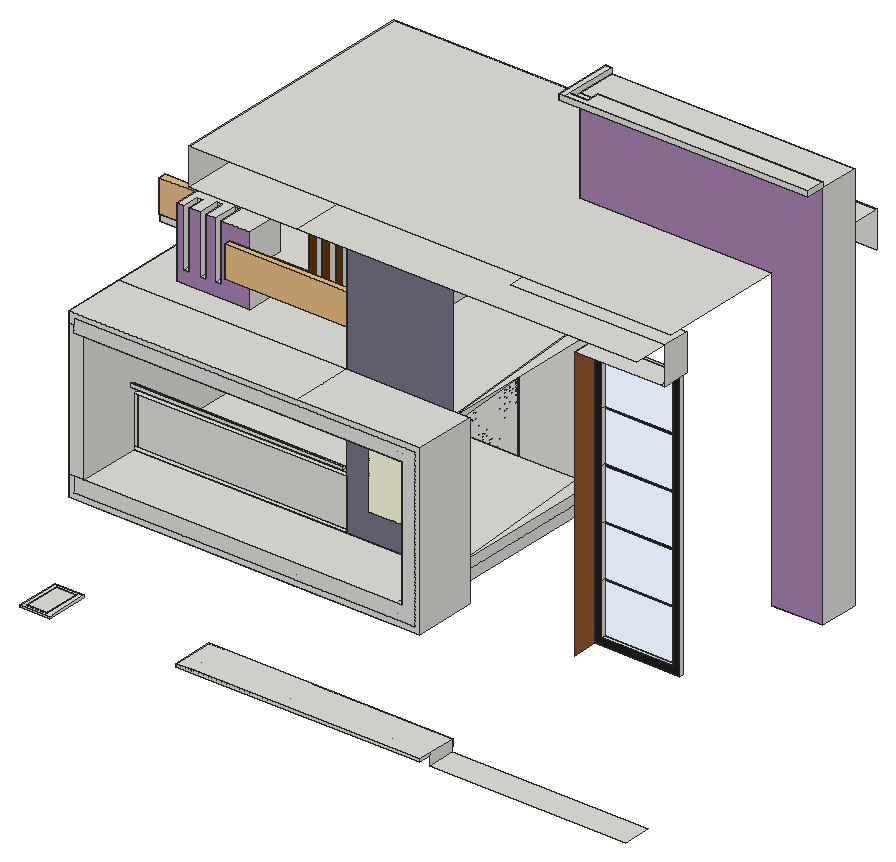
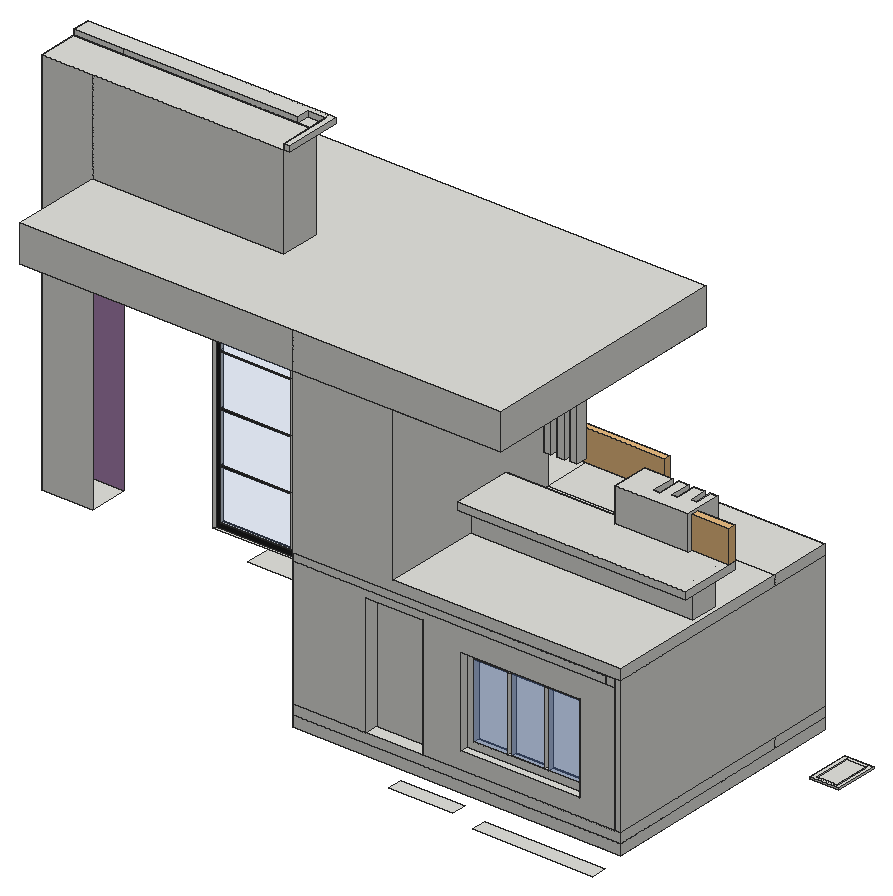
# SketchUp Ruby script. Lengths in inches.
U = 1.inch
M = Sketchup.active_model
def pt(a) = Geom::Point3d.new(a.map { |v| v * U })
def face(e, loops, mat)
  f = e.add_face(loops[0].map { |a| pt(a) })
  loops[1..].each { |l| e.add_face(l.map { |a| pt(a) }).erase! }
  f.material = f.back_material = mat if mat
  f
end
# faces: each face lists its corners as indices into pts; further lists are holes
def faces(e, pts, list, mat = nil) = list.each { |f| face(e, (f[0].is_a?(Array) ? f : [f]).map { |l| l.map { |i| pts[i] } }, mat) }
# xy, xz, yz: faces in a plane at the given z, y or x. An outline is a flat list of corners, or four numbers for a rectangle; further outlines are holes
def ring(l) = l.size == 4 ? [[l[0], l[1]], [l[2], l[1]], [l[2], l[3]], [l[0], l[3]]] : l.each_slice(2).to_a
def flat(e, list, mat, &to3) = list.each { |f| face(e, (f[0].is_a?(Array) ? f : [f]).map { |l| ring(l).map { |u, v| to3.(u, v) } }, mat) }
def xy(e, z, list, mat = nil) = flat(e, list, mat) { |x, y| [x, y, z] }
def xz(e, y, list, mat = nil) = flat(e, list, mat) { |x, z| [x, y, z] }
def yz(e, x, list, mat = nil) = flat(e, list, mat) { |y, z| [x, y, z] }
def lines(e, pts, list) = list.each { |a, b| e.add_line(pt(pts[a]), pt(pts[b])) }
# prism: a flat outline (further loops are holes) pulled along v
def prism(e, loops, v, mat = nil)
  f = face(e, loops, mat); d = Geom::Vector3d.new(v.map { |x| x * U })
  f.pushpull(f.normal.samedirection?(d) ? d.length : -d.length)
end
def box(e, o, s, mat = nil) = prism(e, [[o, [o[0] + s[0], o[1], o[2]], [o[0] + s[0], o[1] + s[1], o[2]], [o[0], o[1] + s[1], o[2]]]], [0, 0, s[2]], mat)
def at(x, y, z, deg = 0) = Geom::Transformation.translation(pt([x, y, z])) * Geom::Transformation.rotation(ORIGIN, Z_AXIS, deg.degrees)
def axes(o, x, y, z) = Geom::Transformation.new([*x, 0, *y, 0, *z, 0, *pt(o).to_a, 1])
def part(name) = M.definitions.add(name)
# library, detail: a bought-in or finely detailed component or shape, given as its bounding box
def library(name, o, s) = part(name).tap { |d| box(d.entities, o, s) }
def detail(e, o, s) = box(e.add_group.entities, o, s)
def put(e, d, t, mat = nil) = e.add_instance(d, t).tap { |i| i.material = mat if mat }
def group(e, t, mat = nil) = e.add_group.tap { |g| g.transformation = t; g.material = mat if mat }.entities
root = M.entities
M.materials.add("Ston e Marble").color = [119, 117, 136]
M.materials.add("[0054_LightYellow]").color = [255, 255, 224]
M.materials.add("[0126_Violet]").color = [168, 130, 177]
M.materials.add("[Color C08]").color = [102, 51, 0]
M.materials.add("[Color L02]").color = [190, 153, 204]
M.materials.add("[Color M08]").color = [30, 30, 30]
M.materials.add("[Translucent Glass Blue]").color = [100, 146, 237]
M.materials["[Translucent Glass Blue]"].alpha = 0.42
M.materials.add("[Translucent Glass Blue]2").color = [100, 149, 237]
M.materials["[Translucent Glass Blue]2"].alpha = 0.01
M.materials.add("[Translucent Glass Blue]3").color = [100, 149, 237]
M.materials["[Translucent Glass Blue]3"].alpha = 0.2
M.materials.add("[Wood Cherry Original]").color = [152, 86, 42]
c1 = part("DOOR12")
g1 = group(c1.entities,at(114.73,28.14,-0.51))
g2 = group(g1,at(0,0,0))
box(g2,[0,0,0],[36,0.5,77.7])
c2 = part("Group\#1")
xy(c2.entities,0,[[0,0,74.375,3.6875]])
xy(c2.entities,4.39,[[4.39,0,24.03,3.6875],[24.03,0,26.53,3.6875],[26.53,0,47.01,3.6875],[47.01,0,49.38,3.6875],[49.38,0,69.98,3.6875]])
xy(c2.entities,50.55,[[4.39,0,24.03,3.6875],[24.03,0,26.53,3.6875],[26.53,0,47.01,3.6875],[47.01,0,49.38,3.6875],[49.38,0,69.98,3.6875]])
xy(c2.entities,54.9375,[[0,0,74.375,3.6875]])
xz(c2.entities,0,[[[0,0,74.375,54.9375],[4.39,4.39,69.98,50.55]],[24.03,4.39,26.53,50.55],[47.01,4.39,49.38,50.55]],"[Color M08]")
xz(c2.entities,3.6875,[[[0,0,74.375,54.9375],[4.39,4.39,69.98,50.55]]])
xz(c2.entities,3.6875,[[4.39,4.39,24.03,50.55],[26.53,4.39,47.01,50.55],[49.38,4.39,69.98,50.55]],"[Translucent Glass Blue]")
yz(c2.entities,0,[[0,0,3.6875,54.9375]])
yz(c2.entities,4.39,[[0,4.39,3.6875,50.55]])
yz(c2.entities,24.03,[[0,4.39,3.6875,50.55]])
yz(c2.entities,26.53,[[0,4.39,3.6875,50.55]])
yz(c2.entities,47.01,[[0,4.39,3.6875,50.55]])
yz(c2.entities,49.38,[[0,4.39,3.6875,50.55]])
yz(c2.entities,69.98,[[0,4.39,3.6875,50.55]])
yz(c2.entities,74.375,[[0,0,3.6875,54.9375]])
c3 = library("Group\#4",[0,0,0],[173.05,8.28,46.41])
xy(root,38.6875,[[252.01,49.71,373.22,66.43]])
xy(root,38.8125,[[165.8,49.71,197.22,67.24]])
xy(root,41.375,[[228.64,66.43,252.01,67.24]])
xy(root,42.6875,[[[4.76,42.32,22.75,69],[7.2,44,19.58,67.25]]])
xy(root,43.9375,[[101.44,41.71,101.44,67.24,110.38,67.24,110.38,49.71,252.01,49.71,252.01,41.71],[[4.76,42.32,22.75,69],[7.2,44,19.58,67.25]],[7.2,44,19.58,67.25]])
xy(root,45.75,[[101.44,41.71,252.01,67.24]])
xy(root,66.45,[[18,233.8,92.38,242.8]])
xy(root,71.33,[[104.9375,233.8,144.61,242.8]])
xy(root,84,[[1.2,84.18,10.2,122.8],[10.2,84.18,10.2,233.8,195.57,233.8,195.57,122.8,142,122.8,142,84.18],[142,84.18,195.57,122.8],[195.57,84.18,204.07,122.8],[204.07,84.18,218.2,122.8],
  [1.2,122.8,10.2,242.8],[195.57,122.8,204.07,233.8],[10.2,233.8,204.07,242.8]])
xy(root,90.65,[[1.2,122.8,204.07,242.8]])
xy(root,90.8125,[[296.76,120.86,349.59,122.8]])
xy(root,95.41,[[301.36,120.86,344.99,122.8]])
xy(root,96.65,[[1.2,84.18,10.42,122.8],[10.42,84.18,204.07,122.8],[1.2,122.8,4.42,122.8,4.42,125.91,10.42,125.91,10.42,233.8,4.42,233.8,4.42,242.8,1.2,242.8],[142,122.8,204.07,122.8,195.57,233.8,10.42,233.8,10.42,125.91,142,125.91],[204.07,122.8,195.57,233.8,204.07,233.8],
  [4.42,233.8,123.41,242.8],[123.41,233.8,159.14,242.8],[159.14,233.8,204.07,242.8]])
xy(root,107.12,[[26.05,233.8,100.42,242.8]])
xy(root,120.43,[[373.22,162.34,404.66,186.78]])
xy(root,128.03,[[4.42,122.8,10.42,125.91],[10.42,122.8,142,125.91]])
xy(root,162.05,[[26.05,233.8,100.42,242.8]])
xy(root,171.64,[[123.41,233.8,159.14,242.8]])
xy(root,176.09,[[10.42,84.18,10.42,233.8,195.57,233.8,204.07,122.8,204.07,84.18],[204.07,84.18,207.2,122.8],[4.42,122.8,10.2,233.8],[10.2,122.8,10.42,233.8],[4.42,233.8,10.2,242.8],
  [10.2,233.8,204.07,242.8]])
xy(root,180.65,[[1.2,84.18,4.42,122.8],[1.2,122.8,4.42,242.8],[4.42,122.8,10.2,242.8],[204.07,122.8,204.07,233.8,195.57,233.8],[10.2,233.8,204.07,242.8]])
xy(root,187.31,[[1.2,84.18,142,122.8],[142,84.18,218.2,122.8],[[1.2,122.8,142,122.8,142,165.79,4.26,165.79,4.26,182.8,142,182.8,142,242.8,1.2,242.8],[23.57,139.58,68.88,162.39]]])
xy(root,194.74,[[28.08,139.58,31.21,149.83]])
xy(root,194.87,[[38.29,139.58,41.54,152.26]])
xy(root,195.12,[[47.72,139.58,51.1,154.2]])
xy(root,204.87,[[0,155.96,4.26,165.79],[4.26,155.96,142,165.79],[0,165.79,4.26,182.8],[0,182.8,4.26,193.76],[4.26,182.8,142,193.76]])
xy(root,209.43,[[0,155.96,142,193.76]])
xy(root,219.41,[[108.41,135.83,113.16,142.39],[115.68,136.58,120.68,143.02],[124.125,136.68,128.8125,142.99]])
xy(root,230.31,[[23.57,139.58,28.08,139.58,28.08,149.83,31.21,149.83,31.21,139.58,38.29,139.58,38.29,152.26,41.54,152.26,41.54,139.58,47.72,139.58,47.72,154.2,51.1,154.2,51.1,139.58,68.88,139.58,68.88,162.39,23.57,162.39]])
xy(root,254.35,[[301.36,120.86,344.99,122.8]])
xy(root,258.95,[[296.76,105.55,349.59,120.86],[349.59,105.55,352.27,122.8],[296.76,120.86,349.59,122.8]])
xy(root,282.04,[[[75.43,84.18,142,242.8],[115.68,136.58,120.68,143.02],[108.41,135.83,113.16,142.39],[124.125,136.68,128.8125,142.99]],[142,84.18,142,122.8,256.63,122.8,256.63,105.55,352.27,105.55,352.27,84.18],[256.63,105.55,352.27,122.8]])
xy(root,304.31,[[75.43,84.18,373.22,84.18,373.22,162.34,254.66,162.34,254.66,186.78,373.22,186.78,373.22,242.8,75.43,242.8]])
xy(root,362.43,[[250.79,150.97,254.66,186.78],[254.66,150.97,404.66,150.97,404.66,162.34,265.51,162.34,265.51,154.47,254.66,154.47],[254.66,154.47,265.51,162.34],[254.66,162.34,404.66,186.78]])
xy(root,365.68,[[250.79,150.97,254.66,186.78],[254.66,150.97,404.66,150.97,404.66,162.34,265.51,162.34,265.51,154.47,254.66,154.47]])
xz(root,41.71,[[101.44,43.9375,110.38,45.75],[110.38,43.9375,252.01,45.75]])
xz(root,42.32,[[4.76,42.6875,22.75,43.9375]])
xz(root,44,[[7.2,42.6875,19.58,43.9375]])
xz(root,49.71,[[197.22,38.5625,228.64,38.5625,228.64,43.9375,165.8,43.9375,165.8,38.8125,197.22,38.8125]],"[Color L02]")
xz(root,67.24,[[165.8,38.8125,165.8,45.75,252.01,45.75,252.01,41.375,197.22,41.375,197.22,38.8125],[101.44,43.9375,110.38,45.75]])
xz(root,67.25,[[7.2,42.6875,19.58,43.9375]])
xz(root,69,[[4.76,42.6875,22.75,43.9375]])
xz(root,84.18,[[1.2,84,218.2,84,218.2,187.31,1.2,187.31,1.2,180.65,4.42,180.65,4.42,184.09,214.98,184.09,214.98,87.22,4.42,87.22,4.42,96.65,1.2,96.65],[4.42,87.22,214.98,87.22,214.98,184.09,4.42,184.09,4.42,176.09,207.2,176.09,207.2,96.59,204.07,96.65,4.42,96.65],[1.2,96.65,10.42,96.65,10.42,176.09,4.42,176.09,4.42,180.65,1.2,180.65]])
xz(root,119.85,[[10.42,132.73,142,134.54]])
xz(root,120.86,[[[296.76,90.8125,349.59,258.95],[301.36,95.41,344.99,254.35]]],"[Color M08]")
xz(root,121.36,[[10.42,132.75,142,134.56]])
xz(root,122.8,[[142,84,204.07,90.65],[204.07,84,218.2,90.65],[1.2,90.65,142,96.65],[142,90.65,204.07,96.65],[204.07,90.65,204.07,96.65,207.2,96.59,218.2,96.4,218.2,90.65],
  [218.2,96.4,207.2,96.59,207.2,180.59,218.2,180.65],[4.42,96.65,10.42,128.03],[4.42,176.09,10.2,180.65]])
xz(root,122.8,[[[207.2,96.59,207.2,176.09,204.07,176.09,204.07,180.65,142,180.65,142,96.65,204.07,96.65],[155.81,113.4,189.18,167.4]],[142,187.31,207.32,282.04]],"Ston e Marble")
xz(root,122.8,[[155.81,113.4,189.18,167.4]],"[0054_LightYellow]")
xz(root,122.8,[[301.36,126.45,344.99,127.2],[301.36,158.24,344.99,158.99],[301.36,190.02,344.99,190.77],[301.36,221.81,344.99,222.56]],"[Color M08]")
xz(root,122.8,[[10.42,96.65,142,128.03]],"[Translucent Glass Blue]2")
xz(root,122.8,[[301.36,95.41,344.99,126.45],[301.36,127.2,344.99,158.24],[301.36,158.99,344.99,190.02],[301.36,190.77,344.99,221.81],[301.36,222.56,344.99,254.35]],"[Translucent Glass Blue]3")
xz(root,125.91,[[4.42,96.65,10.42,128.03],[10.42,96.65,142,128.03]])
xz(root,135.83,[[108.41,219.41,113.16,282.04]],"[Color C08]")
xz(root,136.58,[[115.68,219.41,120.68,282.04]],"[Color C08]")
xz(root,136.68,[[124.125,219.41,128.8125,282.04]],"[Color C08]")
xz(root,139.58,[[23.57,187.31,68.88,187.31,68.88,230.31,51.1,230.31,51.1,195.12,47.72,195.12,47.72,230.31,41.54,230.31,41.54,194.87,38.29,194.87,38.29,230.31,31.21,230.31,31.21,194.74,28.08,194.74,28.08,230.31,23.57,230.31]],"[0126_Violet]")
xz(root,142.39,[[108.41,219.41,113.16,282.04]])
xz(root,142.99,[[124.125,219.41,128.8125,282.04]])
xz(root,143.02,[[115.68,219.41,120.68,282.04]])
xz(root,149.83,[[28.08,194.74,31.21,230.31]])
xz(root,150.97,[[250.79,362.43,404.66,365.68]])
xz(root,152.26,[[38.29,194.87,41.54,230.31]])
xz(root,154.2,[[47.72,195.12,51.1,230.31]])
xz(root,154.47,[[254.66,362.43,265.51,365.68]])
xz(root,155.96,[[0,204.87,142,209.43]])
xz(root,162.34,[[265.51,362.43,373.22,365.68],[373.22,362.43,404.66,365.68]])
xz(root,162.34,[[373.22,120.43,404.66,120.43,404.66,362.43,254.66,362.43,254.66,304.31,373.22,304.31]],"[0126_Violet]")
xz(root,162.39,[[23.57,187.31,68.88,230.31]])
xz(root,165.79,[[4.26,187.31,142,204.87]])
xz(root,182.8,[[4.26,187.31,142,204.87]])
xz(root,186.78,[[373.22,120.43,404.66,362.43],[254.66,304.31,373.22,362.43],[250.79,362.43,254.66,365.68]])
xz(root,193.76,[[0,204.87,142,209.43]])
xz(root,233.8,[[4.42,96.65,10.42,176.09],[[10.42,96.65,123.41,96.65,123.41,171.64,159.14,171.64,159.14,96.65,204.07,96.65,204.07,176.09,10.42,176.09],[26.05,107.12,100.42,162.05]],[123.41,96.65,159.14,171.64],[10.2,176.09,195.57,180.65],[195.57,176.09,204.07,180.65]])
xz(root,242.8,[[1.2,84,204.07,90.65],[1.2,90.65,204.07,96.65],[1.2,96.65,4.42,180.65],[[4.42,96.65,4.42,176.09,204.07,176.09,204.07,96.65,159.14,96.65,159.14,171.64,123.41,171.64,123.41,96.65],[26.05,107.12,100.42,162.05]],[4.42,176.09,10.2,180.65],
  [10.2,176.09,204.07,180.65],[1.2,180.65,1.2,187.31,142,187.31,142,282.04,204.07,282.04,204.07,180.65],[75.43,282.04,204.07,304.31],[204.07,282.04,373.22,304.31]])
yz(root,0,[[155.96,204.87,193.76,209.43]])
yz(root,1.2,[[84.18,84,242.8,90.65],[84.18,90.65,122.8,96.65],[122.8,90.65,242.8,96.65],[84.18,96.65,242.8,180.65],[84.18,180.65,122.8,187.31],
  [122.8,180.65,242.8,187.31]])
yz(root,4.26,[[165.79,187.31,182.8,204.87]])
yz(root,4.42,[[122.8,96.65,125.91,128.03],[233.8,96.65,242.8,176.09],[122.8,176.09,242.8,180.65]])
yz(root,4.76,[[42.32,42.6875,69,43.9375]])
yz(root,7.2,[[44,42.6875,67.25,43.9375]])
yz(root,10.2,[[122.8,176.09,233.8,180.65],[233.8,176.09,242.8,180.65]])
yz(root,10.42,[[[84.18,96.65,122.8,96.65,122.8,128.03,125.91,128.03,125.91,96.65,233.8,96.65,233.8,176.09,84.18,176.09],[119.85,132.73,119.85,134.54,121.36,134.56,121.36,132.75]]])
yz(root,19.58,[[44,42.6875,67.25,43.9375]])
yz(root,22.75,[[42.32,42.6875,69,43.9375]])
yz(root,23.57,[[139.58,187.31,162.39,230.31]])
yz(root,26.05,[[233.8,107.12,242.8,162.05]])
yz(root,28.08,[[139.58,194.74,149.83,230.31]])
yz(root,31.21,[[139.58,194.74,149.83,230.31]])
yz(root,38.29,[[139.58,194.87,152.26,230.31]])
yz(root,41.54,[[139.58,194.87,152.26,230.31]])
yz(root,47.72,[[139.58,195.12,154.2,230.31]])
yz(root,51.1,[[139.58,195.12,154.2,230.31]])
yz(root,68.88,[[139.58,187.31,162.39,230.31]])
yz(root,75.43,[[84.18,282.04,242.8,304.31]])
yz(root,100.42,[[233.8,107.12,242.8,162.05]])
yz(root,101.44,[[41.71,43.9375,67.24,45.75]])
yz(root,108.41,[[135.83,219.41,142.39,282.04]])
yz(root,113.16,[[135.83,219.41,142.39,282.04]])
yz(root,115.68,[[136.58,219.41,143.02,282.04]])
yz(root,120.68,[[136.58,219.41,143.02,282.04]])
yz(root,123.41,[[233.8,96.65,242.8,171.64]])
yz(root,124.125,[[136.68,219.41,142.99,282.04]])
yz(root,128.8125,[[136.68,219.41,142.99,282.04]])
yz(root,142,[[122.8,96.65,125.91,128.03],[119.85,132.73,121.36,132.75,121.36,134.56,119.85,134.54],[122.8,187.31,122.8,282.04,242.8,282.04,242.8,187.31,182.8,187.31,182.8,204.87,193.76,204.87,193.76,209.43,155.96,209.43,155.96,204.87,165.79,204.87,165.79,187.31],[155.96,204.87,165.79,209.43],[182.8,204.87,193.76,209.43]])
yz(root,159.14,[[233.8,96.65,242.8,171.64]])
yz(root,197.22,[[49.71,38.5625,49.71,38.8125,51.27,38.8125],[49.71,38.5625,51.27,38.8125,67.24,41.375,67.24,38.8125,49.71,38.8125]])
yz(root,204.07,[[122.8,84,242.8,90.65],[122.8,90.65,242.8,96.65],[233.8,96.65,242.8,176.09],[233.8,176.09,242.8,180.65]])
yz(root,207.2,[[84.18,96.59,122.8,176.09]])
yz(root,218.2,[[84.18,84,122.8,187.31]])
yz(root,228.64,[[49.71,38.5625,66.43,41.24,66.43,41.375],[66.43,41.24,67.24,41.375,66.43,41.375]])
yz(root,250.79,[[150.97,362.43,186.78,365.68]])
yz(root,252.01,[[49.71,38.6875,66.43,45.75],[66.43,41.375,67.24,45.75],[41.71,43.9375,49.71,45.75]])
yz(root,254.66,[[162.34,304.31,186.78,362.43],[154.47,362.43,186.78,365.68]])
yz(root,265.51,[[154.47,362.43,162.34,365.68]])
yz(root,296.76,[[120.86,90.8125,122.8,258.95]])
yz(root,296.76,[[105.55,90.8125,120.86,258.95]],"[Wood Cherry Original]")
yz(root,301.36,[[120.86,95.41,122.8,127.2],[120.86,127.2,122.8,158.99],[120.86,158.99,122.8,190.77],[120.86,190.77,122.8,222.56],[120.86,222.56,122.8,254.35]])
yz(root,344.99,[[120.86,95.41,122.8,127.2],[120.86,127.2,122.8,158.99],[120.86,158.99,122.8,190.77],[120.86,190.77,122.8,222.56],[120.86,222.56,122.8,254.35]])
yz(root,349.59,[[120.86,90.8125,122.8,258.95]])
yz(root,352.27,[[105.55,258.95,122.8,282.04]])
yz(root,404.66,[[162.34,120.43,186.78,362.43],[150.97,362.43,162.34,365.68]])
p = [[197.22,49.71,38.5625],[228.64,49.71,38.5625],[228.64,66.43,41.24],[228.64,67.24,41.375],[197.22,67.24,41.375],[197.22,51.27,38.8125],
  [207.2,122.8,96.59],[204.07,122.8,96.65],[204.07,84.18,96.65],[207.2,84.18,96.59],[142,119.85,132.73],[10.42,119.85,132.73],
  [10.42,121.36,132.75],[142,121.36,132.75],[142,121.36,134.56],[10.42,121.36,134.56],[10.42,119.85,134.54],[142,119.85,134.54],
  [195.57,233.8,180.65],[204.07,122.8,180.65],[204.07,122.8,176.09],[195.57,233.8,176.09],[142,122.8,180.65],[142,122.8,187.31],
  [4.26,182.8,209.43],[4.26,182.8,204.87],[4.26,165.79,209.43],[4.26,165.79,204.87],[204.07,122.8,90.65],[204.07,84.18,90.65],
  [142,122.8,90.65],[142,84.18,90.65],[204.07,84.18,180.65],[207.2,122.8,180.59],[207.2,84.18,180.59],[228.64,49.71,45.75],
  [228.64,49.71,43.9375],[228.64,66.43,45.75],[228.64,66.43,41.375],[110.38,49.71,43.9375],[110.38,49.71,45.75],[165.8,49.71,43.9375],
  [165.8,49.71,45.75]]
faces(root,p,[[0,1,2,3,4,5],[6,7,8,9],[10,11,12,13],[14,15,16,17],[18,19,20,21]])
lines(root,p,[[22,23],[24,25],[26,27],[28,29],[30,31],[19,32],[33,34],[35,36],[37,38],[39,40],[41,42]])
put(root,c1,at(8.6875,205.66,97.16))
put(root,c2,at(26.05,233.8,107.12))
put(root,c3,axes([0.09,155.28,209.43],[0.21615,0,0],[0,0.56703,0],[0,0,0.42913]))
put(root,c3,axes([66.6875,126.33,210.9],[0.4352,0,0],[0,-0.4383,0],[0,0,0.41808]))
